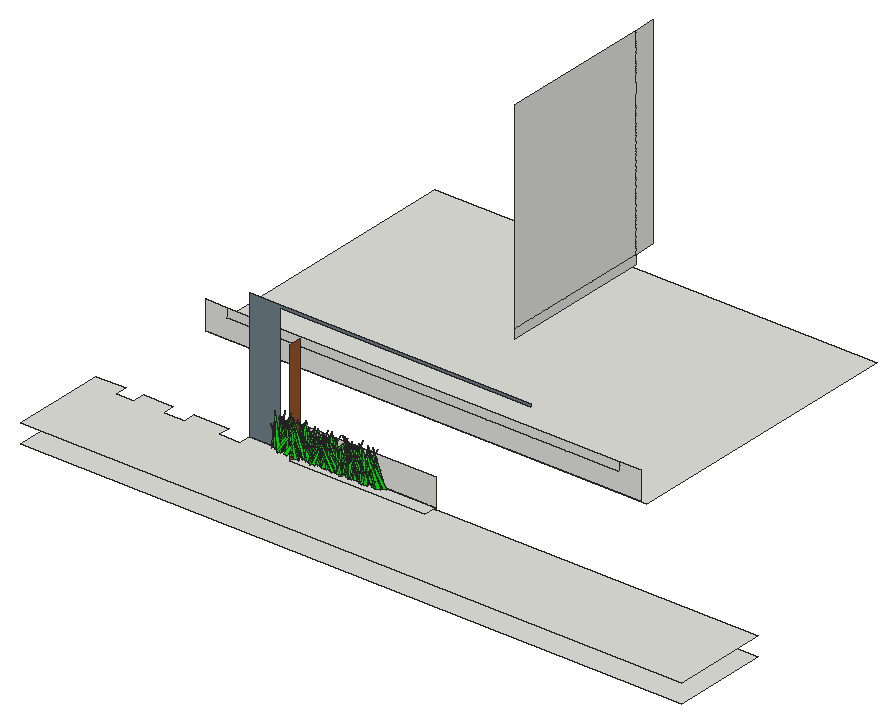
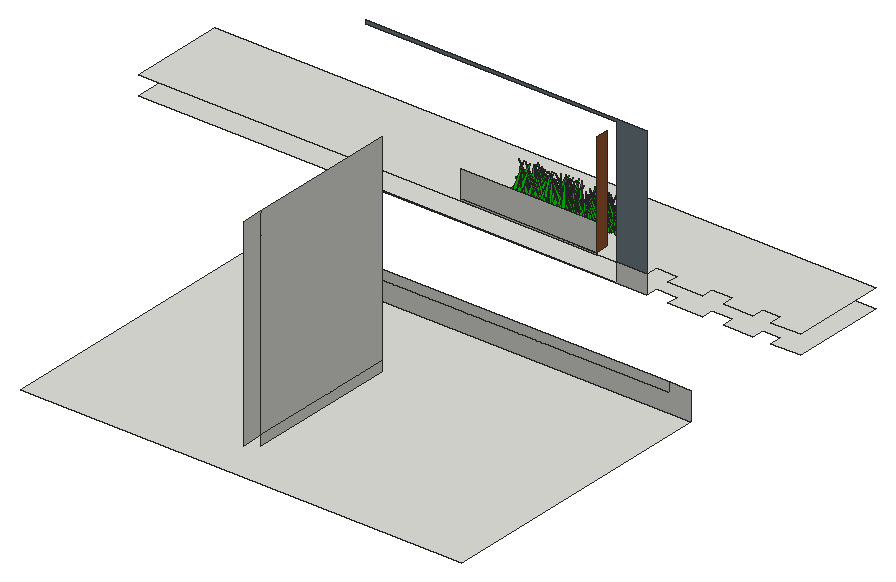
# SketchUp Ruby script. Lengths in inches.
U = 1.inch
M = Sketchup.active_model
def pt(a) = Geom::Point3d.new(a.map { |v| v * U })
def face(e, loops, mat)
  f = e.add_face(loops[0].map { |a| pt(a) })
  loops[1..].each { |l| e.add_face(l.map { |a| pt(a) }).erase! }
  f.material = f.back_material = mat if mat
  f
end
# faces: each face lists its corners as indices into pts; further lists are holes
def faces(e, pts, list, mat = nil) = list.each { |f| face(e, (f[0].is_a?(Array) ? f : [f]).map { |l| l.map { |i| pts[i] } }, mat) }
# xy, xz, yz: faces in a plane at the given z, y or x. An outline is a flat list of corners, or four numbers for a rectangle; further outlines are holes
def ring(l) = l.size == 4 ? [[l[0], l[1]], [l[2], l[1]], [l[2], l[3]], [l[0], l[3]]] : l.each_slice(2).to_a
def flat(e, list, mat, &to3) = list.each { |f| face(e, (f[0].is_a?(Array) ? f : [f]).map { |l| ring(l).map { |u, v| to3.(u, v) } }, mat) }
def xy(e, z, list, mat = nil) = flat(e, list, mat) { |x, y| [x, y, z] }
def xz(e, y, list, mat = nil) = flat(e, list, mat) { |x, z| [x, y, z] }
def yz(e, x, list, mat = nil) = flat(e, list, mat) { |y, z| [x, y, z] }
def lines(e, pts, list) = list.each { |a, b| e.add_line(pt(pts[a]), pt(pts[b])) }
# prism: a flat outline (further loops are holes) pulled along v
def prism(e, loops, v, mat = nil)
  f = face(e, loops, mat); d = Geom::Vector3d.new(v.map { |x| x * U })
  f.pushpull(f.normal.samedirection?(d) ? d.length : -d.length)
end
def box(e, o, s, mat = nil) = prism(e, [[o, [o[0] + s[0], o[1], o[2]], [o[0] + s[0], o[1] + s[1], o[2]], [o[0], o[1] + s[1], o[2]]]], [0, 0, s[2]], mat)
def at(x, y, z, deg = 0) = Geom::Transformation.translation(pt([x, y, z])) * Geom::Transformation.rotation(ORIGIN, Z_AXIS, deg.degrees)
def axes(o, x, y, z) = Geom::Transformation.new([*x, 0, *y, 0, *z, 0, *pt(o).to_a, 1])
def part(name) = M.definitions.add(name)
# library, detail: a bought-in or finely detailed component or shape, given as its bounding box
def library(name, o, s) = part(name).tap { |d| box(d.entities, o, s) }
def detail(e, o, s) = box(e.add_group.entities, o, s)
def put(e, d, t, mat = nil) = e.add_instance(d, t).tap { |i| i.material = mat if mat }
def group(e, t, mat = nil) = e.add_group.tap { |g| g.transformation = t; g.material = mat if mat }.entities
root = M.entities
M.materials.add("[0065_Lime]").color = [0, 255, 0]
M.materials.add("[0111_SlateGray]1").color = [112, 128, 136]
M.materials.add("[Wood Cherry Original]").color = [152, 86, 42]
c1 = part("fur_instance\#9")
p = [[0.8125,0,1.79],[0.67,-0.02,1.48],[0,-0.11,0],[0,0.11,0]]
faces(c1.entities,p,[[0,1,2,3]])
xy(root,-11.8125,[[5.71,0,5.71,39.75,18.06,39.75,18.06,34.8125,25.54,34.8125,25.54,39.75,37.97,39.75,37.97,34.8125,46.56,34.8125,46.56,39.75,61.07,39.75,61.07,34.8125,69.9,34.8125,69.9,39.75,282.96,39.75,282.96,0],[5.71,97.05,190.59,217.05]])
xy(root,-3.9375,[[5.71,0,282.96,0,282.96,39.75,69.9,39.75,69.9,34.8125,61.07,34.8125,61.07,39.75,46.56,39.75,46.56,34.8125,37.97,34.8125,37.97,39.75,25.54,39.75,25.54,34.8125,18.06,34.8125,18.06,39.75,5.71,39.75]])
xy(root,-3.22,[[90.86,34.4375,147.74,39.75]])
xz(root,39.75,[[69.9,-11.8125,187.77,-11.8125,187.77,-11.6,82.49,-11.6,82.49,-3.9375,69.9,-3.9375],[90.86,-3.9375,147.74,-3.22],[90.86,-3.22,147.74,8.21]])
xz(root,39.75,[[69.9,-3.9375,82.49,-3.9375,82.49,48.65,187.77,48.65,187.77,49.9375,69.9,49.9375]],"[0111_SlateGray]1")
xz(root,97.05,[[5.71,-11.8125,5.71,0,14.71,0,14.71,-3.9375,179.21,-3.9375,179.21,0,187.77,0,187.77,-11.8125],[14.71,-3.9375,179.21,0]])
yz(root,90.86,[[34.4375,-3.22,39.75,40.28]],"[Wood Cherry Original]")
yz(root,96.96,[[144.8,-3.9375,208.05,0],[144.8,0,208.05,84],[208.05,0,217.05,84]])
put(root,c1,axes([92.79,29.98,1.48],[-0.58333,0.77098,1.02112],[-4.97072,-0.15376,2.01136],[2.64037,-0.11914,4.01216]),"[0065_Lime]")
put(root,c1,axes([103.32,29.88,1.48],[7.1029,0.31919,1.31566],[-1.75091,0.99455,-1.83096],[-2.17034,0.24227,5.78292]),"[0065_Lime]")
put(root,c1,axes([125.77,30.55,1.48],[-1.70264,-0.61512,0.00015],[4.2331,-0.23136,-0.97332],[1.11527,-0.06093,3.69456]),"[0065_Lime]")
put(root,c1,axes([95.11,30.57,1.48],[5.31195,-0.36314,1.56137],[1.84145,0.76964,1.85306],[-2.64051,-0.1938,4.43333]),"[0065_Lime]")
put(root,c1,axes([98.1,30,1.48],[-4.04751,0.15641,0.10165],[-0.99331,-0.53165,1.24305],[0.51763,0.20281,3.18023]),"[0065_Lime]")
put(root,c1,axes([89.75,30.17,1.48],[3.36043,1.10546,2.70946],[-8.16205,0.56399,-1.01285],[-2.52336,-0.3521,6.88442]),"[0065_Lime]")
put(root,c1,axes([114.3,30.59,1.48],[-1.95357,-0.5869,0.46036],[3.7659,-0.28242,-1.49098],[1.89284,-0.04385,3.44153]),"[0065_Lime]")
put(root,c1,axes([89.24,30.06,1.48],[7.55138,-0.34583,0.38796],[2.43715,0.9629,-2.62465],[0.58731,0.45084,5.90321]),"[0065_Lime]")
put(root,c1,axes([129.5,30.63,1.48],[-3.8626,-0.35547,0.32293],[2.33158,-0.52997,-1.0962],[1.05874,-0.12977,3.59222]),"[0065_Lime]")
put(root,c1,axes([115.48,30.75,1.48],[-8.62051,0.11947,1.34027],[-1.40948,-1.13764,-2.6001],[1.20466,-0.47614,6.54877]),"[0065_Lime]")
put(root,c1,axes([92.9,30.62,1.48],[6.38662,0.44092,3.10801],[-4.19935,0.9467,1.20909],[-2.60976,-0.44432,5.66039]),"[0065_Lime]")
put(root,c1,axes([124.37,30.25,1.48],[4.27088,-0.13396,1.05245],[1.33671,0.58269,-1.10372],[-0.89228,0.23171,3.38405]),"[0065_Lime]")
put(root,c1,axes([123.4,30.9,1.48],[5.70529,-0.41584,0.72311],[2.36392,0.75631,2.23368],[-1.98992,-0.29379,4.72671]),"[0065_Lime]")
put(root,c1,axes([112.07,30.6,1.48],[-6.7851,0.30696,0.49718],[-2.26828,-0.91524,-1.54642],[-0.02403,-0.28059,5.58806]),"[0065_Lime]")
put(root,c1,axes([118.5625,30.35,1.48],[5.18025,0.14407,2.08085],[-0.58396,0.80534,-0.90652],[-2.6934,0.10248,4.19867]),"[0065_Lime]")
put(root,c1,axes([125.17,30.8,1.48],[-0.32984,-0.99586,0.68507],[6.88837,-0.01342,1.54046],[-1.86733,0.12639,5.56159]),"[0065_Lime]")
put(root,c1,axes([102.23,30.83,1.48],[8.25978,-0.22003,0.48181],[1.42357,1.14359,1.35299],[-0.88104,-0.21501,6.7031]),"[0065_Lime]")
put(root,c1,axes([114.1875,30.97,1.48],[2.809,-0.88134,0.28444],[6.08472,0.39512,1.2657],[-1.56118,-0.04581,5.44489]),"[0065_Lime]")
put(root,c1,axes([97.18,29.95,1.48],[3.67515,1.10396,0.03245],[-7.09681,0.46914,-3.01287],[-3.37036,0.21595,6.37945]),"[0065_Lime]")
put(root,c1,axes([130.86,30.99,1.48],[0.37993,-1.16417,0.65259],[7.90764,0.08571,2.07759],[-2.59836,0.09062,6.41819]),"[0065_Lime]")
put(root,c1,axes([111.9,30.72,1.48],[-3.62105,-0.76784,0.04709],[4.88876,-0.45081,2.41052],[-2.44187,0.23608,4.75616]),"[0065_Lime]")
put(root,c1,axes([110.89,30.87,1.48],[-6.27926,-0.60083,1.51065],[4.09984,-0.92013,-0.98757],[2.21882,-0.00017,6.09994]),"[0065_Lime]")
put(root,c1,axes([95.75,30.63,1.48],[-3.97898,0.90399,1.84724],[-6.82232,-0.5272,-1.07792],[-0.00062,-0.36947,6.05776]),"[0065_Lime]")
put(root,c1,axes([118.12,30.67,1.48],[-3.11738,-0.77601,2.98113],[5.95806,-0.57743,-0.91443],[2.90378,0.35168,5.07668]),"[0065_Lime]")
put(root,c1,axes([123.4,30.75,1.48],[-5.54614,-0.73165,0.29941],[5.09664,-0.74275,1.64508],[-1.12718,0.24156,5.96516]),"[0065_Lime]")
put(root,c1,axes([102.05,30.6875,1.48],[5.09356,0.67925,0.76887],[-4.88699,0.6731,1.49475],[0.61466,-0.27723,5.51291]),"[0065_Lime]")
put(root,c1,axes([97.12,30.6,1.48],[-7.78946,0.69891,0.00051],[-4.93715,-1.08647,-0.91198],[-0.60287,-0.13283,7.46205]),"[0065_Lime]")
put(root,c1,axes([118.05,30.94,1.48],[7.6876,0.2306,1.77998],[-2.106,1.08435,1.31075],[-1.74542,-0.29269,6.25829]),"[0065_Lime]")
put(root,c1,axes([104.02,30.54,1.48],[1.58733,0.88723,0.50831],[-6.21464,0.19917,1.19153],[1.27872,-0.13339,5.1599]),"[0065_Lime]")
put(root,c1,axes([104.33,30.6875,1.48],[-6.06924,-0.38858,0.35704],[2.75405,-0.80193,1.72953],[-0.50491,0.29671,5.14201]),"[0065_Lime]")
put(root,c1,axes([100.19,31.125,1.48],[-7.42553,-0.45359,1.8752],[2.70548,-1.08192,-1.68097],[2.90082,-0.15203,6.36792]),"[0065_Lime]")
put(root,c1,axes([119.01,31.27,1.48],[-5.98064,-0.79454,2.08447],[4.66459,-0.90508,-2.7053],[4.09641,-0.12938,6.1238]),"[0065_Lime]")
put(root,c1,axes([121.29,31.18,1.48],[1.81968,-0.89398,0.50761],[6.16084,0.26958,1.29625],[-1.70551,0.01998,5.22405]),"[0065_Lime]")
put(root,c1,axes([94.72,30.58,1.48],[1.40549,0.95642,0.99325],[-6.67698,0.23325,-1.27469],[-1.7988,-0.1185,5.50762]),"[0065_Lime]")
put(root,c1,axes([106.99,31.23,1.48],[7.32784,-0.28176,0.44385],[1.77492,0.99478,1.77238],[-1.08078,-0.2767,5.92007]),"[0065_Lime]")
put(root,c1,axes([119.1,30.5,1.48],[7.92996,0.67818,0.81449],[-4.66016,1.11837,-1.18401],[-1.60593,0.10349,7.45767]),"[0065_Lime]")
put(root,c1,axes([109.3125,30.625,1.48],[-6.44069,0.37009,1.36204],[-2.26285,-0.92535,1.34549],[2.14943,0.13478,5.49779]),"[0065_Lime]")
put(root,c1,axes([113.39,31.56,1.48],[6.06915,-0.9786,0.12428],[6.46017,0.80137,2.71009],[-2.60575,-0.29253,7.00832]),"[0065_Lime]")
put(root,c1,axes([107.58,31.24,1.48],[-3.35986,-0.5665,0.88734],[3.45143,-0.48739,-1.77996],[2.35174,-0.09404,3.88001]),"[0065_Lime]")
put(root,c1,axes([111.67,31.125,1.48],[1.2371,-1.11758,2.03928],[7.99277,0.26047,1.57517],[-2.37817,0.29407,6.35478]),"[0065_Lime]")
put(root,c1,axes([114.09,30.87,1.48],[-3.98834,0.88371,0.82926],[-6.10856,-0.4824,-2.21237],[-1.81006,-0.31922,5.63905]),"[0065_Lime]")
put(root,c1,axes([126.2,30.53,1.48],[2.43439,1.15064,0.8346],[-7.91486,0.36809,-1.73016],[-2.33668,-0.04806,6.72994]),"[0065_Lime]")
put(root,c1,axes([107.92,30.85,1.48],[2.46239,-0.54126,1.976],[4.54965,0.30927,-0.91248],[-0.19811,0.37496,3.60501]),"[0065_Lime]")
put(root,c1,axes([106.91,30.96,1.48],[6.04361,-0.57406,0.14582],[3.90744,0.79744,-1.95444],[1.20578,0.29312,5.60263]),"[0065_Lime]")
put(root,c1,axes([113.97,31.45,1.48],[5.38693,-0.60437,0.33817],[3.99294,0.73192,1.74754],[-1.65162,-0.20171,5.32782]),"[0065_Lime]")
put(root,c1,axes([98.89,31.14,1.48],[-2.32904,-0.53619,0.30624],[3.69808,-0.29776,1.13898],[-1.01315,0.14576,3.45334]),"[0065_Lime]")
put(root,c1,axes([88.79,30.9,1.48],[3.69867,1.07428,0.58376],[-7.30802,0.45811,2.38656],[2.35727,-0.26538,6.48288]),"[0065_Lime]")
put(root,c1,axes([113.76,31.21,1.48],[-5.38182,0.26664,0.16691],[-1.8681,-0.7182,-1.40743],[-0.39133,-0.23858,4.42328]),"[0065_Lime]")
put(root,c1,axes([87.0625,31.4,1.48],[-4.93179,-0.5442,1.24066],[3.47273,-0.72116,-1.46616],[2.29464,-0.07823,4.88539]),"[0065_Lime]")
put(root,c1,axes([115.52,30.7,1.48],[-0.18701,1.06111,0.09285],[-7.09702,-0.01921,-2.10317],[-2.58246,-0.02406,5.77314]),"[0065_Lime]")
put(root,c1,axes([101.59,31.375,1.48],[0.488,-1.19903,1.65508],[8.46145,0.13988,1.74492],[-2.31399,0.25862,6.72959]),"[0065_Lime]")
put(root,c1,axes([128.52,31.26,1.48],[-5.31797,-1.02482,0.77342],[7.13821,-0.67943,2.30674],[-1.77225,0.33857,6.97021]),"[0065_Lime]")
put(root,c1,axes([112.32,31.41,1.48],[7.30887,0.20638,0.38435],[-1.54046,0.95833,2.13891],[0.0856,-0.37522,5.67423]),"[0065_Lime]")
put(root,c1,axes([106.76,31.14,1.48],[2.38613,0.90155,1.91759],[-6.81001,0.2834,1.14202],[0.58748,-0.37662,5.44964]),"[0065_Lime]")
put(root,c1,axes([107.47,31.45,1.48],[5.2142,-0.31984,0.25352],[2.14359,0.7164,1.11484],[-0.82638,-0.15977,4.49149]),"[0065_Lime]")
put(root,c1,axes([89.61,31.26,1.48],[-0.8928,-0.67018,1.60691],[4.77255,-0.21454,-1.2439],[1.96789,0.21626,3.74574]),"[0065_Lime]")
put(root,c1,axes([125.49,30.91,1.48],[-4.85426,0.90999,1.86804],[-6.06831,-0.7531,1.85987],[3.22312,-0.04738,6.31507]),"[0065_Lime]")
put(root,c1,axes([85.77,31.67,1.48],[6.38989,-0.08617,1.68738],[-0.4511,0.836,2.56079],[-2.11563,-0.43851,4.55043]),"[0065_Lime]")
put(root,c1,axes([95.51,31.1875,1.48],[-2.62377,0.77683,0.47222],[-4.70275,-0.26211,-2.83983],[-2.96379,-0.27181,4.08802]),"[0065_Lime]")
put(root,c1,axes([108.45,31.03,1.48],[-6.3388,0.4697,1.5409],[-3.08558,-0.92833,1.08382],[2.2893,0.0493,5.72738]),"[0065_Lime]")
put(root,c1,axes([122.74,31.57,1.48],[-2.98246,-0.60613,0.30947],[4.14979,-0.41861,-1.01311],[1.23734,-0.05708,4.14368]),"[0065_Lime]")
put(root,c1,axes([105.51,31.38,1.48],[-2.13972,-0.61605,0.42286],[4.03645,-0.2401,1.79261],[-1.78831,0.19516,3.5402]),"[0065_Lime]")
put(root,c1,axes([109.18,31.7,1.48],[2.30908,-1.23827,1.50257],[8.45064,0.39053,2.19202],[-3.10716,0.14192,7.07833]),"[0065_Lime]")
put(root,c1,axes([90.03,31.66,1.48],[-5.06251,-0.7403,1.03674],[5.02171,-0.73282,-1.31003],[2.04021,-0.03321,5.797]),"[0065_Lime]")
put(root,c1,axes([115.8,30.88,1.48],[6.65928,0.5648,0.54523],[-3.63263,0.90458,-2.04394],[-1.84639,0.25735,5.98773]),"[0065_Lime]")
put(root,c1,axes([93.36,31.71,1.48],[-4.77478,-0.6892,0.75398],[4.61404,-0.67817,-1.43947],[1.90421,-0.08489,5.37856]),"[0065_Lime]")
put(root,c1,axes([107.07,31.24,1.48],[-5.96904,-0.31842,1.90546],[2.77851,-0.85619,0.96451],[1.70366,0.28072,5.10305]),"[0065_Lime]")
put(root,c1,axes([107.73,31.62,1.48],[-1.00996,-1.10787,1.2127],[7.79461,-0.08534,1.68253],[-1.90458,0.23821,6.24276]),"[0065_Lime]")
put(root,c1,axes([125.625,31.47,1.48],[-6.06816,0.74028,0.52365],[-4.9943,-0.74995,-2.76612],[-1.79609,-0.41572,5.92245]),"[0065_Lime]")
put(root,c1,axes([88.94,31.54,1.48],[-5.4149,0.21049,0.89083],[-1.74786,-0.73799,-1.18624],[0.6232,-0.24085,4.41335]),"[0065_Lime]")
put(root,c1,axes([100.22,31.7,1.48],[-3.09754,-0.59087,1.17267],[3.60067,-0.4783,-1.78286],[2.60681,-0.04145,3.856]),"[0065_Lime]")
put(root,c1,axes([112.2,31.46,1.48],[-0.80099,0.62312,1.97642],[-4.60215,-0.23305,1.2281],[2.09492,-0.27373,3.45357]),"[0065_Lime]")
put(root,c1,axes([115.14,31.29,1.48],[-5.21069,0.22736,1.14146],[-1.34647,-0.7511,0.94636],[1.6656,0.10408,4.336]),"[0065_Lime]")
put(root,c1,axes([86.97,31.54,1.48],[8.60553,0.54138,0.66615],[-3.93858,1.1858,1.37167],[-0.04376,-0.26335,7.5457]),"[0065_Lime]")
put(root,c1,axes([91.78,31.28,1.48],[-3.53028,0.28561,0.40698],[-1.73344,-0.47617,1.24867],[1.17334,0.15585,3.06923]),"[0065_Lime]")
put(root,c1,axes([107.65,31.37,1.48],[0.24892,0.63787,0.61826],[-4.42701,0.06244,-0.97951],[-1.25922,-0.09344,3.56588]),"[0065_Lime]")
put(root,c1,axes([122.62,31.15,1.48],[3.55505,1.14732,0.94601],[-8.0893,0.51975,-1.00906],[-1.6068,-0.0782,7.17306]),"[0065_Lime]")
put(root,c1,axes([129.51,31.47,1.48],[-4.14605,0.56445,0.40944],[-4.02475,-0.56378,-0.92131],[-0.43665,-0.163,4.60443]),"[0065_Lime]")
put(root,c1,axes([97.42,32,1.48],[0.80257,-1.15425,0.52555],[7.94177,0.13267,1.73942],[-2.19548,0.05796,6.48417]),"[0065_Lime]")
put(root,c1,axes([93.97,31.33,1.48],[-0.6566,0.96219,0.82919],[-6.57471,-0.13173,1.67733],[2.16792,-0.10807,5.33802]),"[0065_Lime]")
put(root,c1,axes([120.94,32,1.48],[-5.88219,-0.57547,1.26661],[3.58903,-0.84296,-1.80571],[2.51311,-0.1431,5.54341]),"[0065_Lime]")
put(root,c1,axes([105.16,31.9,1.48],[-8.16822,0.1186,2.69486],[-1.6157,-1.19652,-1.47566],[3.01299,-0.3201,6.51447]),"[0065_Lime]")
put(root,c1,axes([112.69,31.8,1.48],[-3.23902,-0.72831,0.33317],[4.96621,-0.41332,1.66865],[-1.53909,0.19908,4.68311]),"[0065_Lime]")
put(root,c1,axes([109.8,31.21,1.48],[-6.3745,0.5211,0.54272],[-3.18475,-0.84359,2.39209],[2.01373,0.31541,5.50113]),"[0065_Lime]")
put(root,c1,axes([116.99,31.7,1.48],[4.60601,0.49139,0.51868],[-3.54866,0.62712,0.94177],[0.20677,-0.18345,4.60883]),"[0065_Lime]")
put(root,c1,axes([121.6,32.18,1.48],[4.2606,-0.71787,0.06027],[4.87915,0.57568,1.5577],[-1.51623,-0.1647,5.18196]),"[0065_Lime]")
put(root,c1,axes([127.5,31.35,1.48],[-5.44543,0.40537,1.60311],[-1.90481,-0.77439,2.28048],[2.92882,0.25004,4.46375]),"[0065_Lime]")
put(root,c1,axes([96.89,31.42,1.48],[-6.73005,0.47729,0.79189],[-3.13787,-0.94262,1.39301],[1.62442,0.15659,5.97169]),"[0065_Lime]")
put(root,c1,axes([112.52,32.16,1.48],[6.08545,-0.87769,2.12109],[5.55385,0.92914,2.34052],[-3.86893,-0.04674,6.69609]),"[0065_Lime]")
put(root,c1,axes([99.12,31.92,1.48],[-8.09997,0.50342,1.67392],[-3.99133,-1.11787,-1.5133],[1.06744,-0.35981,7.04359]),"[0065_Lime]")
put(root,c1,axes([101.09,32.12,1.48],[1.63004,-0.65308,0.06866],[4.45826,0.2232,1.11101],[-1.31592,-0.05278,3.84909]),"[0065_Lime]")
put(root,c1,axes([103.1,31.48,1.48],[-3.80488,0.26386,0.05314],[-1.58052,-0.46069,1.77473],[1.01593,0.27148,2.96005]),"[0065_Lime]")
put(root,c1,axes([106.71,31.8,1.48],[5.78676,-0.46555,1.03714],[3.52416,0.79462,-1.05764],[-0.42754,0.24874,5.31978]),"[0065_Lime]")
put(root,c1,axes([110.2,31.8,1.48],[4.8299,-0.61215,2.05657],[4.95839,0.66443,-1.0776],[-0.88611,0.38127,5.17981]),"[0065_Lime]")
put(root,c1,axes([108.4,32.16,1.48],[-8.08492,0.06373,1.68597],[-1.00565,-1.12543,-1.76525],[1.86828,-0.33,6.34577]),"[0065_Lime]")
put(root,c1,axes([93.66,31.6875,1.48],[7.62464,0.2447,0.46949],[-1.63397,1.06343,-1.0151],[-0.83411,0.15359,6.28017]),"[0065_Lime]")
put(root,c1,axes([106.01,32.55,1.48],[-5.02127,-1.01568,0.68454],[6.60582,-0.69647,-2.56752],[3.05235,-0.16355,6.68264]),"[0065_Lime]")
put(root,c1,axes([121.28,31.92,1.48],[-1.2514,0.81002,1.0691],[-5.7095,-0.11652,-1.46349],[-1.53582,-0.22683,4.56951]),"[0065_Lime]")
put(root,c1,axes([93.04,31.49,1.48],[-7.40628,0.30981,0.14477],[-1.87946,-0.92749,2.89269],[1.16637,0.47274,5.58047]),"[0065_Lime]")
put(root,c1,axes([107.72,31.9,1.48],[4.49685,0.92819,0.21821],[-6.26513,0.58379,2.21482],[2.11014,-0.24473,6.1109]),"[0065_Lime]")
put(root,c1,axes([121.03,32.32,1.48],[1.90491,-1.06094,1.59785],[7.41674,0.33441,1.59009],[-2.41999,0.18977,6.13104]),"[0065_Lime]")
put(root,c1,axes([132.5,32.43,1.48],[-1.61142,-1.22637,0.75009],[8.12292,-0.15854,2.8599],[-3.32237,0.20719,6.62842]),"[0065_Lime]")
put(root,c1,axes([110.66,32.18,1.48],[4.70116,-0.96348,0.56153],[6.17536,0.53687,-3.33981],[3.05861,0.39695,5.88002]),"[0065_Lime]")
put(root,c1,axes([108.94,31.76,1.48],[3.4773,0.83104,0.7525],[-5.37342,0.4996,-2.0593],[-2.63795,0.07779,5.18667]),"[0065_Lime]")
put(root,c1,axes([104,31.92,1.48],[8.76318,0.15614,1.04788],[-0.87165,1.22777,-1.30749],[-1.46103,0.20405,7.0652]),"[0065_Lime]")
put(root,c1,axes([114.49,32.42,1.48],[-7.17968,-0.34985,1.38155],[2.21691,-1.03075,-1.1237],[2.04176,-0.11104,6.07822]),"[0065_Lime]")
put(root,c1,axes([88.1,31.91,1.48],[1.33378,0.6779,0.43655],[-4.41481,0.20193,-1.58256],[-2.01774,0.0063,3.7512]),"[0065_Lime]")
put(root,c1,axes([121.65,31.94,1.48],[-9.19537,-0.04376,0.69793],[0.51379,-1.25697,1.83808],[0.75445,0.32268,7.25469]),"[0065_Lime]")
put(root,c1,axes([123.48,32.14,1.48],[5.77881,0.96701,1.20032],[-7.00204,0.76272,1.71402],[0.71282,-0.34733,7.10578]),"[0065_Lime]")
put(root,c1,axes([125.56,32.43,1.48],[2.38446,-0.92224,0.8852],[6.56537,0.29996,-1.22931],[1.0748,0.21371,5.54534]),"[0065_Lime]")
put(root,c1,axes([127.59,31.87,1.48],[3.82719,0.82954,0.62049],[-5.60831,0.54522,-1.53744],[-1.99499,0.05869,5.5124]),"[0065_Lime]")
put(root,c1,axes([94.8125,32.27,1.48],[3.92119,0.49276,0.84934],[-3.65888,0.52837,0.90468],[-0.00485,-0.21436,4.18223]),"[0065_Lime]")
put(root,c1,axes([126.79,32.13,1.48],[1.16982,0.6332,0.392],[-4.1811,0.12381,1.55375],[1.74832,-0.12758,3.45349]),"[0065_Lime]")
put(root,c1,axes([115.68,32.44,1.48],[6.97325,0.29247,0.2401],[-2.0757,0.9352,1.71456],[0.33264,-0.29541,5.66565]),"[0065_Lime]")
put(root,c1,axes([98.96,32.09,1.48],[-7.24741,-0.17317,0.70738],[1.44584,-0.96845,1.85664],[0.42966,0.33787,5.68422]),"[0065_Lime]")
put(root,c1,axes([102.17,32.25,1.48],[-1.32535,0.6788,1.7114],[-4.70479,-0.28971,1.43977],[2.37217,-0.19534,3.81169]),"[0065_Lime]")
put(root,c1,axes([98.87,32.06,1.48],[4.76294,0.35076,0.02287],[-2.39329,0.64402,-1.20205],[-0.70995,0.18216,4.20566]),"[0065_Lime]")
put(root,c1,axes([115.17,32.5625,1.48],[-3.95108,-1.06249,1.01867],[7.60687,-0.51945,1.36651],[-0.93626,0.26341,6.80363]),"[0065_Lime]")
put(root,c1,axes([127.03,32.36,1.48],[-3.88725,-0.45636,0.28434],[3.1365,-0.50016,1.47159],[-0.91214,0.22497,3.84849]),"[0065_Lime]")
put(root,c1,axes([100.93,32.16,1.48],[-7.31201,-0.29669,0.23953],[2.06902,-0.95202,2.27565],[-0.5136,0.38865,5.75724]),"[0065_Lime]")
put(root,c1,axes([97.89,32.67,1.48],[1.82244,-0.98741,0.42767],[6.90559,0.23507,-1.28351],[1.40256,0.12561,5.76373]),"[0065_Lime]")
put(root,c1,axes([109.52,32.08,1.48],[-4.86915,0.74744,1.2509],[-5.01666,-0.7173,1.44186],[2.34343,0.01746,5.68576]),"[0065_Lime]")
put(root,c1,axes([108.19,32.68,1.48],[-2.87913,-0.64251,1.08085],[4.30204,-0.44452,-1.27252],[2.04098,0.03061,4.20696]),"[0065_Lime]")
put(root,c1,axes([93.93,32.91,1.48],[-8.56417,-0.13357,0.90225],[0.47513,-1.13128,-2.62796],[1.38136,-0.43899,6.49767]),"[0065_Lime]")
put(root,c1,axes([106.66,32.375,1.48],[8.11406,0.60402,0.20094],[-4.29157,1.12859,0.97992],[0.34776,-0.16575,7.40448]),"[0065_Lime]")
put(root,c1,axes([110.01,32.1,1.48],[5.48472,0.54011,0.36769],[-3.56353,0.74775,-1.63595],[-1.50997,0.19719,5.19641]),"[0065_Lime]")
put(root,c1,axes([110.75,32.44,1.48],[0.49241,0.58397,1.1297],[-4.11527,-0.00581,1.2875],[1.50487,-0.20698,3.15121]),"[0065_Lime]")
put(root,c1,axes([98.6875,32.3,1.48],[-3.76542,0.79536,1.41216],[-5.48884,-0.57734,1.2126],[2.21921,-0.07842,5.39522]),"[0065_Lime]")
put(root,c1,axes([88.06,32.3,1.48],[-6.06907,0.23155,2.09754],[-0.95357,-0.90783,1.53263],[2.90787,0.18557,4.8804]),"[0065_Lime]")
put(root,c1,axes([88.86,32.63,1.48],[7.47869,0.55774,1.62264],[-4.33008,1.03784,1.25077],[-0.99216,-0.32531,6.7724]),"[0065_Lime]")
put(root,c1,axes([107.38,32.61,1.48],[3.64579,0.31876,0.58656],[-2.38009,0.48553,0.94652],[0.03401,-0.1923,3.36204]),"[0065_Lime]")
put(root,c1,axes([120.35,32.41,1.48],[-8.41983,-0.44458,1.35091],[3.50836,-1.1419,1.87526],[0.67809,0.38772,7.07196]),"[0065_Lime]")
put(root,c1,axes([127.64,32.34,1.48],[3.88733,0.3454,0.48161],[-2.24193,0.54144,-1.03873],[-1.16887,0.1102,3.59401]),"[0065_Lime]")
put(root,c1,axes([87.16,32.8,1.48],[3.21831,-1.03881,0.83381],[7.24394,0.397,-1.92568],[1.79699,0.2601,6.2694]),"[0065_Lime]")
put(root,c1,axes([89.93,32.69,1.48],[3.51757,-0.74543,0.12966],[4.645,0.41941,-2.57943],[2.56734,0.26251,4.48921]),"[0065_Lime]")
put(root,c1,axes([108.89,32.47,1.48],[-4.84003,-0.37415,1.81309],[3.39933,-0.62022,1.71523],[0.70905,0.41949,4.15312]),"[0065_Lime]")
put(root,c1,axes([96.02,32.75,1.48],[-2.66642,-0.97294,3.29124],[7.37478,-0.53287,-1.32537],[3.15054,0.42391,5.88792]),"[0065_Lime]")
put(root,c1,axes([120.62,33.05,1.48],[0.80783,-0.95648,0.83012],[6.35801,0.159,2.04522],[-2.63625,0.09038,5.18695]),"[0065_Lime]")
put(root,c1,axes([116.5,32.73,1.48],[0.93498,0.65636,1.90109],[-4.86853,0.23034,-1.08062],[-1.89153,-0.26844,3.72107]),"[0065_Lime]")
put(root,c1,axes([87.54,32.46,1.48],[-1.84613,1.25452,1.98976],[-8.47409,-0.3701,2.61707],[3.72566,-0.22016,6.93854]),"[0065_Lime]")
put(root,c1,axes([111.27,32.83,1.48],[2.32961,-0.51013,0.7907],[3.73102,0.29461,-0.90407],[0.45162,0.19754,3.39021]),"[0065_Lime]")
put(root,c1,axes([118.66,33.14,1.48],[2.83883,-0.52253,0.29526],[3.22806,0.37527,1.71906],[-1.8814,-0.14457,3.39504]),"[0065_Lime]")
put(root,c1,axes([102.36,32.55,1.48],[-3.21263,1.03867,0.73493],[-7.39643,-0.42902,-1.07505],[-0.86444,-0.18935,6.46713]),"[0065_Lime]")
put(root,c1,axes([109.98,33.05,1.48],[-5.97114,-0.007,0.50723],[-0.16038,-0.79571,-1.61741],[0.60466,-0.28023,4.57996]),"[0065_Lime]")
put(root,c1,axes([120.26,33.38,1.48],[5.42261,-1.03752,0.9086],[6.69213,0.76124,2.70232],[-3.31368,-0.16048,6.94433]),"[0065_Lime]")
put(root,c1,axes([121.93,32.68,1.48],[0.34911,0.71932,1.06987],[-5.02175,0.10291,-1.23424],[-1.64828,-0.16117,3.98691]),"[0065_Lime]")
put(root,c1,axes([131.39,32.94,1.48],[-5.73893,-0.90496,1.48908],[6.68663,-0.79192,0.92369],[0.34064,0.2989,6.95559]),"[0065_Lime]")
put(root,c1,axes([121.91,32.58,1.48],[-0.16448,1.06331,0.96335],[-7.22373,0.03379,-2.06585],[-2.54578,-0.16458,5.79967]),"[0065_Lime]")
put(root,c1,axes([91.88,32.51,1.48],[-7.16997,0.34958,0.08244],[-2.39172,-0.97906,1.48686],[0.69218,0.23815,5.99151]),"[0065_Lime]")
put(root,c1,axes([99.5,33.46,1.48],[5.94772,-0.40865,0.57624],[2.0012,0.70756,3.14768],[-2.2259,-0.4558,4.36965]),"[0065_Lime]")
put(root,c1,axes([101.15,32.6,1.48],[-4.60465,0.34743,0.59087],[-2.13873,-0.63181,1.42118],[1.43766,0.17287,4.00671]),"[0065_Lime]")
put(root,c1,axes([94.03,32.99,1.48],[4.49477,0.5376,1.43697],[-4.21098,0.58674,1.35947],[-0.15943,-0.34099,4.60471]),"[0065_Lime]")
put(root,c1,axes([109.22,33.125,1.48],[4.77119,-1.1271,0.49361],[7.75749,0.6185,-2.28874],[2.12757,0.27243,7.23819]),"[0065_Lime]")
put(root,c1,axes([123.65,33.09,1.48],[-0.47232,-1.03594,1.57151],[7.12062,0.03697,2.23271],[-2.7167,0.27702,5.57885]),"[0065_Lime]")
put(root,c1,axes([97.92,32.97,1.48],[-4.21308,0.82213,1.42286],[-5.93002,-0.4795,-2.33376],[-1.45805,-0.42542,5.38019]),"[0065_Lime]")
put(root,c1,axes([90.78,32.99,1.48],[-1.46921,-0.49976,1.47789],[3.54142,-0.28878,-0.9429],[1.84627,0.15623,2.98469]),"[0065_Lime]")
put(root,c1,axes([127.8,32.72,1.48],[-4.1925,0.02457,1.77082],[0.58654,-0.62514,1.20946],[2.1038,0.22326,3.19173]),"[0065_Lime]")
put(root,c1,axes([99.55,32.6,1.48],[-3.75665,0.8458,0.91222],[-5.79952,-0.55083,1.31161],[1.96314,-0.00873,5.62038]),"[0065_Lime]")
put(root,c1,axes([97.05,32.71,1.48],[5.4933,-0.50017,1.88218],[4.23737,0.6788,-2.1381],[-0.26239,0.4907,4.8762]),"[0065_Lime]")
put(root,c1,axes([109.6,33.22,1.48],[5.28233,0.06808,0.8181],[-0.85296,0.68709,1.72796],[-0.72025,-0.31438,3.95364]),"[0065_Lime]")
put(root,c1,axes([100.09,32.82,1.48],[5.18457,-0.10997,0.93912],[1.14745,0.69131,-1.47871],[-0.79296,0.28135,4.00042]),"[0065_Lime]")
put(root,c1,axes([93.77,33.375,1.48],[4.73866,-0.4552,0.62488],[2.89164,0.65579,1.49911],[-1.64998,-0.158,4.42187]),"[0065_Lime]")
put(root,c1,axes([91.875,32.93,1.48],[-2.70647,0.52883,0.0481],[-3.65467,-0.36678,-0.93528],[-0.90013,-0.10088,3.65278]),"[0065_Lime]")
put(root,c1,axes([118.87,32.99,1.48],[2.18837,0.97228,2.62922],[-7.2037,0.41969,-1.23354],[-2.53603,-0.35315,5.77271]),"[0065_Lime]")
put(root,c1,axes([113.67,33.41,1.48],[-7.25286,-0.38783,0.08458],[2.69372,-1.00234,-1.17685],[0.61009,-0.18492,6.20162]),"[0065_Lime]")
put(root,c1,axes([106.1,32.79,1.48],[5.82773,0.34807,0.06432],[-2.36408,0.78927,-1.401],[-0.74384,0.21857,4.9566]),"[0065_Lime]")
put(root,c1,axes([103.02,33.03,1.48],[3.88921,0.90254,0.51432],[-6.13304,0.48452,2.19426],[2.01006,-0.26796,5.69991]),"[0065_Lime]")
put(root,c1,axes([118.7,33.33,1.48],[7.5357,0.28627,0.43539],[-2.10505,1.01363,1.77408],[0.07439,-0.31539,6.09681]),"[0065_Lime]")
put(root,c1,axes([113.24,32.95,1.48],[1.05699,0.83114,1.17865],[-5.65371,0.21072,-1.62453],[-2.26281,-0.13826,4.60952]),"[0065_Lime]")
put(root,c1,axes([121.67,33.01,1.48],[7.17344,-0.10559,0.40126],[0.86109,0.96719,-1.6568],[-0.25795,0.29225,5.6281]),"[0065_Lime]")
put(root,c1,axes([111.57,33.36,1.48],[4.99946,-0.44787,2.45182],[3.02563,0.81703,0.91907],[-3.17646,0.07333,4.73436]),"[0065_Lime]")
put(root,c1,axes([103.87,33.34,1.48],[-1.71747,-0.60022,0.75295],[4.29211,-0.20525,0.99495],[-0.82468,0.18175,3.61022]),"[0065_Lime]")
put(root,c1,axes([105.21,32.89,1.48],[5.36045,0.72007,0.84899],[-4.80964,0.76127,-1.54344],[-2.05346,0.09666,5.83132]),"[0065_Lime]")
put(root,c1,axes([98.02,33.41,1.48],[-4.4148,-0.82139,0.65038],[5.84375,-0.58947,1.29936],[-0.812,0.22358,5.81509]),"[0065_Lime]")
put(root,c1,axes([105,33.2,1.48],[2.25086,0.84666,0.87743],[-5.87534,0.25354,1.77445],[1.71697,-0.24235,4.92176]),"[0065_Lime]")
put(root,c1,axes([116.34,32.97,1.48],[1.51057,0.98626,0.56139],[-6.85075,0.22876,-1.27021],[-1.6754,-0.04616,5.70009]),"[0065_Lime]")
put(root,c1,axes([117.24,33.39,1.48],[7.13284,0.77712,1.48486],[-5.81607,0.97156,1.44677],[-0.30242,-0.35561,7.19766]),"[0065_Lime]")
put(root,c1,axes([88.65,33.11,1.48],[7.96371,0.42755,2.20617],[-2.45925,1.17108,-1.73136],[-3.25056,0.16148,6.71487]),"[0065_Lime]")
put(root,c1,axes([127.67,33.24,1.48],[2.16593,0.50308,0.76656],[-3.18586,0.33143,-1.33263],[-1.88574,0.01789,3.13188]),"[0065_Lime]")
put(root,c1,axes([94.17,33.38,1.48],[2.35495,0.97584,1.40584],[-6.79848,0.2252,2.29681],[2.23513,-0.34317,5.50487]),"[0065_Lime]")
put(root,c1,axes([103.8,33.44,1.48],[4.08942,0.58849,0.50053],[-4.2028,0.55014,1.0449],[0.50474,-0.18716,4.64521]),"[0065_Lime]")
put(root,c1,axes([91.15,33.4375,1.48],[5.33237,-0.77902,2.11049],[6.11645,0.69679,-1.60652],[-0.2361,0.457,6.04712]),"[0065_Lime]")
put(root,c1,axes([101.79,33.37,1.48],[-5.14767,0.25375,1.12159],[-1.4038,-0.7325,1.29019],[1.78648,0.15556,4.24564]),"[0065_Lime]")
put(root,c1,axes([93.41,33.09,1.48],[9.06492,0.22021,0.76627],[-1.06717,1.18079,-3.0178],[-1.48476,0.49576,6.84738]),"[0065_Lime]")
put(root,c1,axes([129.53,33.23,1.48],[0.53111,1.23528,0.65479],[-8.15626,0.11202,-2.70391],[-3.37689,-0.07627,6.63379]),"[0065_Lime]")
put(root,c1,axes([120.16,33.29,1.48],[2.283,0.70562,0.35032],[-4.36257,0.30994,-2.10808],[-2.5238,0.10255,3.96087]),"[0065_Lime]")
put(root,c1,axes([106.98,33.26,1.48],[-5.71812,0.29677,0.34465],[-1.70054,-0.7256,2.26886],[1.32215,0.35022,4.40875]),"[0065_Lime]")
put(root,c1,axes([110.41,33.25,1.48],[1.22447,1.19079,0.41028],[-8.37916,0.18103,-1.0599],[-1.36316,-0.0431,6.88359]),"[0065_Lime]")
put(root,c1,axes([125,33.47,1.48],[1.60766,0.85696,0.32236],[-5.67107,0.23065,-1.83327],[-2.278,0.03059,4.79143]),"[0065_Lime]")
